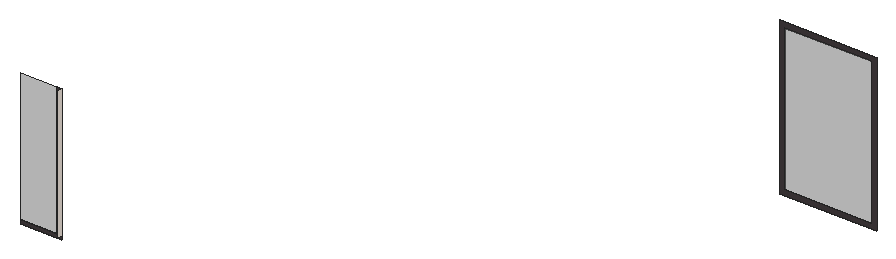
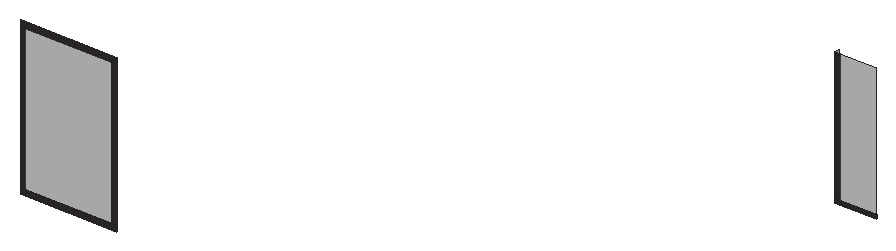
# SketchUp Ruby script. Lengths in inches.
U = 1.inch
M = Sketchup.active_model
def pt(a) = Geom::Point3d.new(a.map { |v| v * U })
def face(e, loops, mat)
  f = e.add_face(loops[0].map { |a| pt(a) })
  loops[1..].each { |l| e.add_face(l.map { |a| pt(a) }).erase! }
  f.material = f.back_material = mat if mat
  f
end
# faces: each face lists its corners as indices into pts; further lists are holes
def faces(e, pts, list, mat = nil) = list.each { |f| face(e, (f[0].is_a?(Array) ? f : [f]).map { |l| l.map { |i| pts[i] } }, mat) }
# xy, xz, yz: faces in a plane at the given z, y or x. An outline is a flat list of corners, or four numbers for a rectangle; further outlines are holes
def ring(l) = l.size == 4 ? [[l[0], l[1]], [l[2], l[1]], [l[2], l[3]], [l[0], l[3]]] : l.each_slice(2).to_a
def flat(e, list, mat, &to3) = list.each { |f| face(e, (f[0].is_a?(Array) ? f : [f]).map { |l| ring(l).map { |u, v| to3.(u, v) } }, mat) }
def xy(e, z, list, mat = nil) = flat(e, list, mat) { |x, y| [x, y, z] }
def xz(e, y, list, mat = nil) = flat(e, list, mat) { |x, z| [x, y, z] }
def yz(e, x, list, mat = nil) = flat(e, list, mat) { |y, z| [x, y, z] }
def lines(e, pts, list) = list.each { |a, b| e.add_line(pt(pts[a]), pt(pts[b])) }
# prism: a flat outline (further loops are holes) pulled along v
def prism(e, loops, v, mat = nil)
  f = face(e, loops, mat); d = Geom::Vector3d.new(v.map { |x| x * U })
  f.pushpull(f.normal.samedirection?(d) ? d.length : -d.length)
end
def box(e, o, s, mat = nil) = prism(e, [[o, [o[0] + s[0], o[1], o[2]], [o[0] + s[0], o[1] + s[1], o[2]], [o[0], o[1] + s[1], o[2]]]], [0, 0, s[2]], mat)
def at(x, y, z, deg = 0) = Geom::Transformation.translation(pt([x, y, z])) * Geom::Transformation.rotation(ORIGIN, Z_AXIS, deg.degrees)
def axes(o, x, y, z) = Geom::Transformation.new([*x, 0, *y, 0, *z, 0, *pt(o).to_a, 1])
def part(name) = M.definitions.add(name)
# library, detail: a bought-in or finely detailed component or shape, given as its bounding box
def library(name, o, s) = part(name).tap { |d| box(d.entities, o, s) }
def detail(e, o, s) = box(e.add_group.entities, o, s)
def put(e, d, t, mat = nil) = e.add_instance(d, t).tap { |i| i.material = mat if mat }
def group(e, t, mat = nil) = e.add_group.tap { |g| g.transformation = t; g.material = mat if mat }.entities
root = M.entities
M.materials.add("[0009_Linen]").color = [250, 240, 230]
M.materials.add("[Asphalt New]").color = [67, 60, 62]
M.materials.add("[Translucent Glass Gray]").color = [128, 128, 128]
M.materials["[Translucent Glass Gray]"].alpha = 0.5
xz(root,304.24,[[288.77,52.25,323.93,55.45],[323.93,52.25,328.15,55.45],[323.93,55.45,328.15,181.51]],"[Asphalt New]")
xz(root,304.24,[[288.77,55.45,323.93,181.51]],"[Translucent Glass Gray]")
xz(root,683.93,[[[711.72,59.63,803.59,208.29],[716.4,64.3125,798.91,203.6]]],"[Asphalt New]")
xz(root,683.93,[[716.4,64.3125,798.91,203.6]],"[Translucent Glass Gray]")
yz(root,328.15,[[300.43,55.45,304.24,181.51]],"[0009_Linen]")
